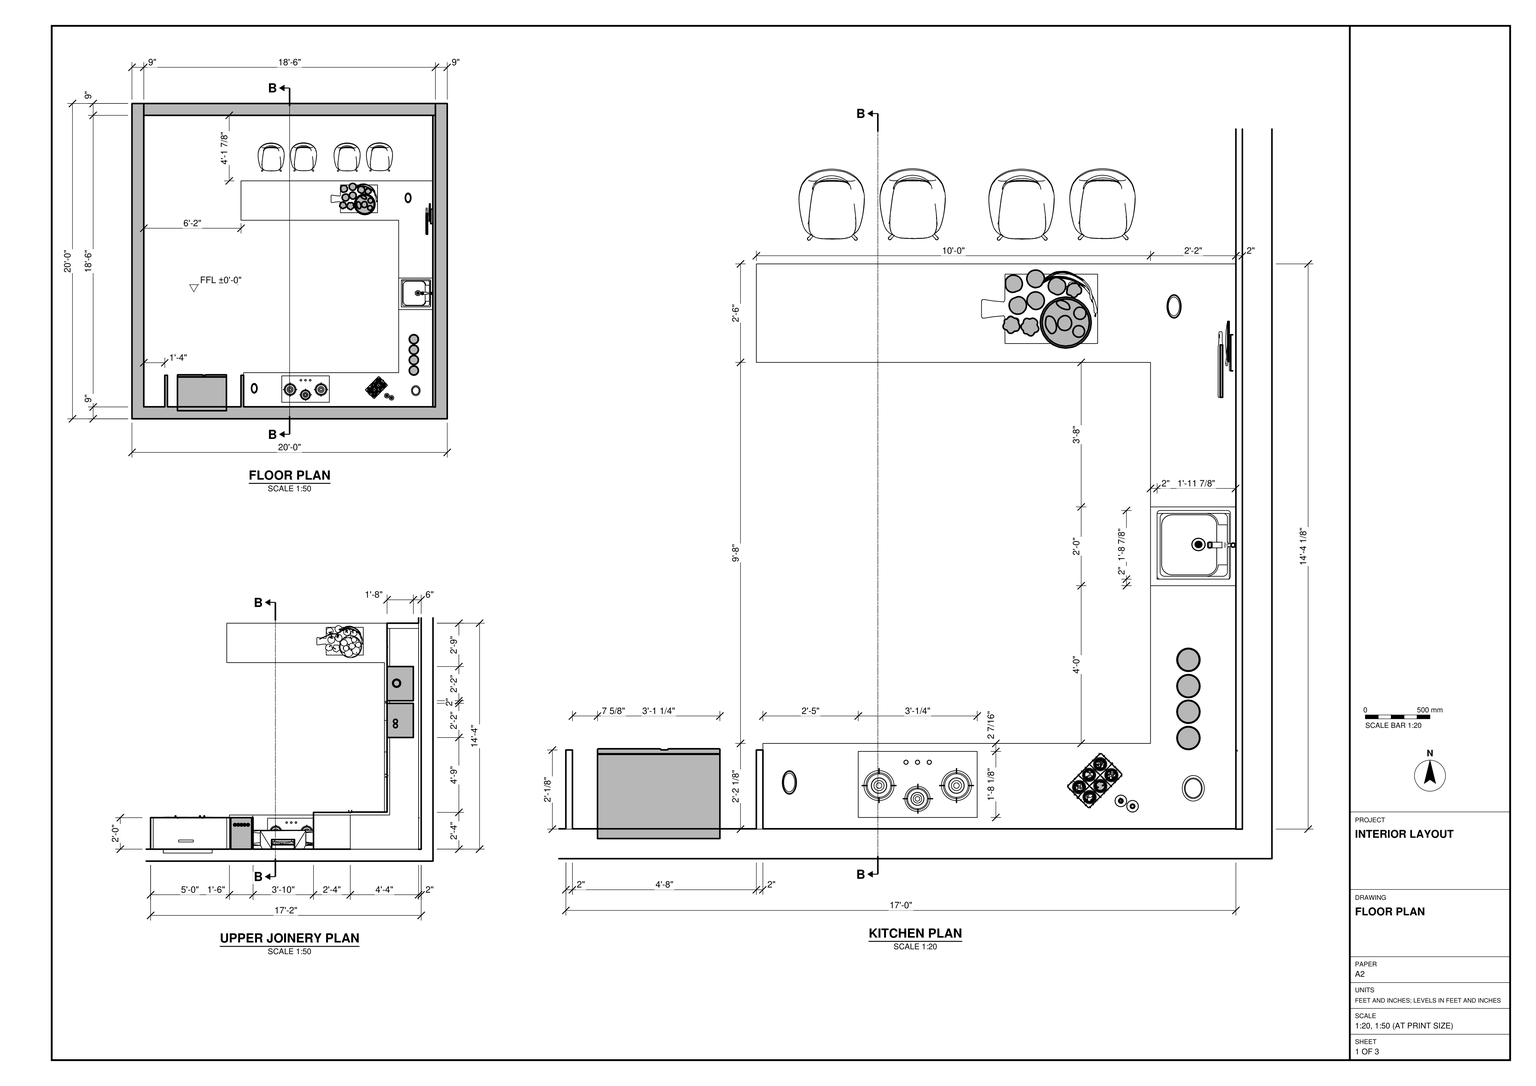
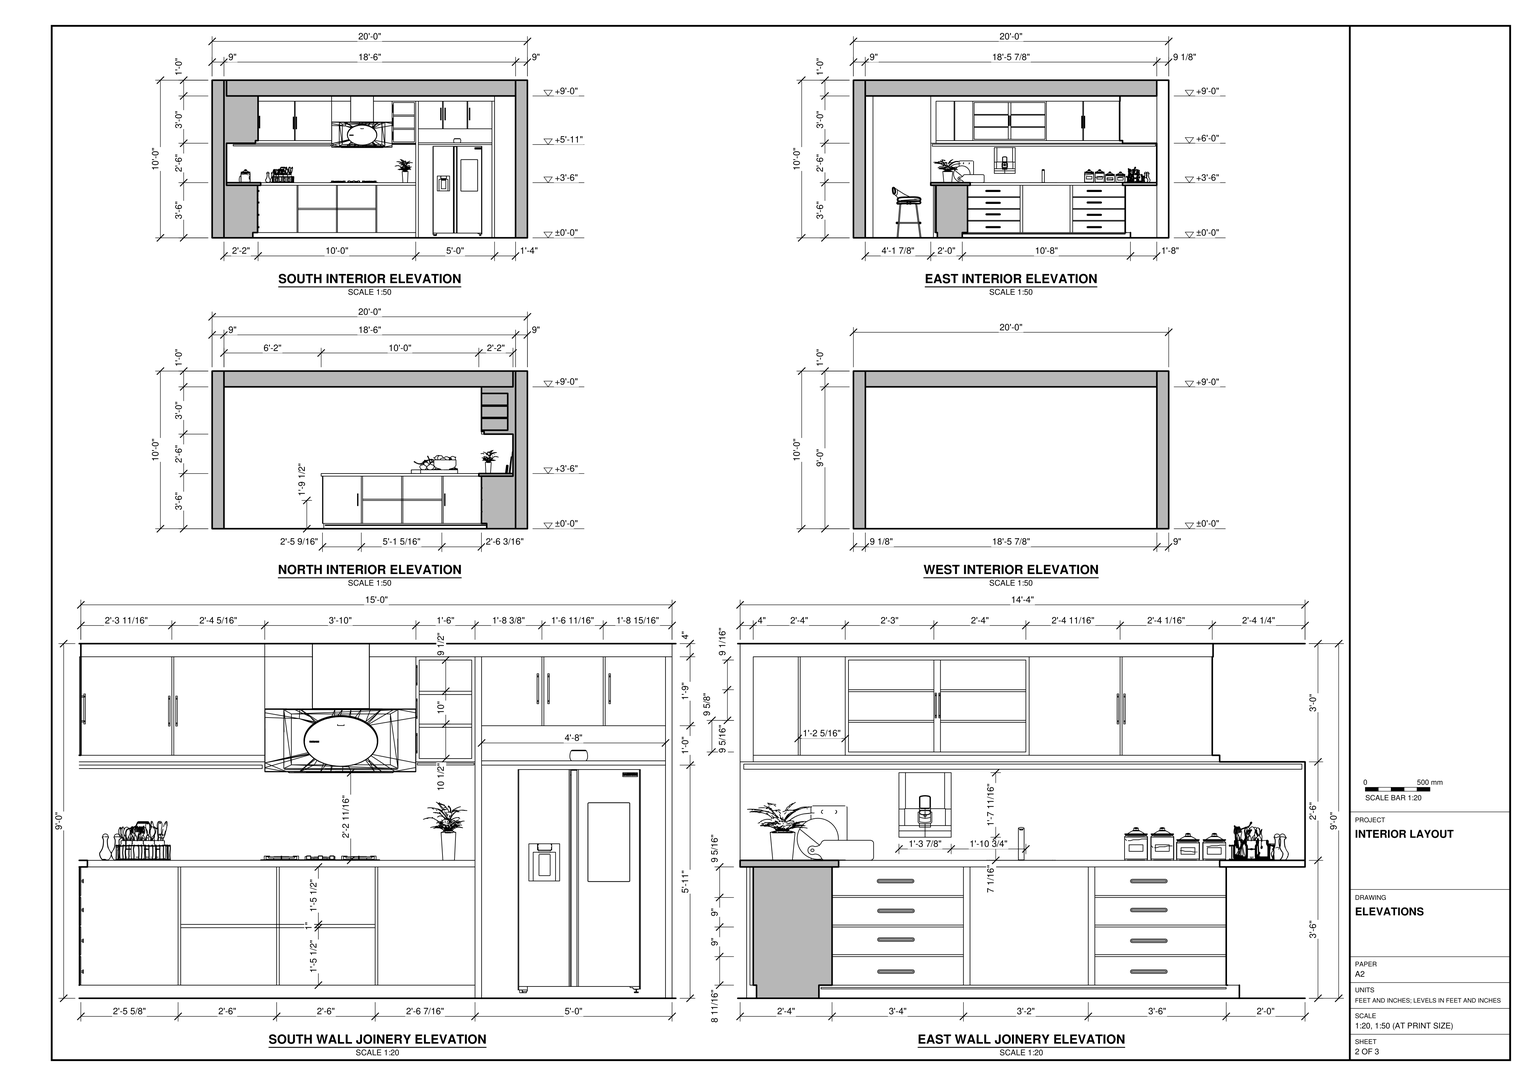
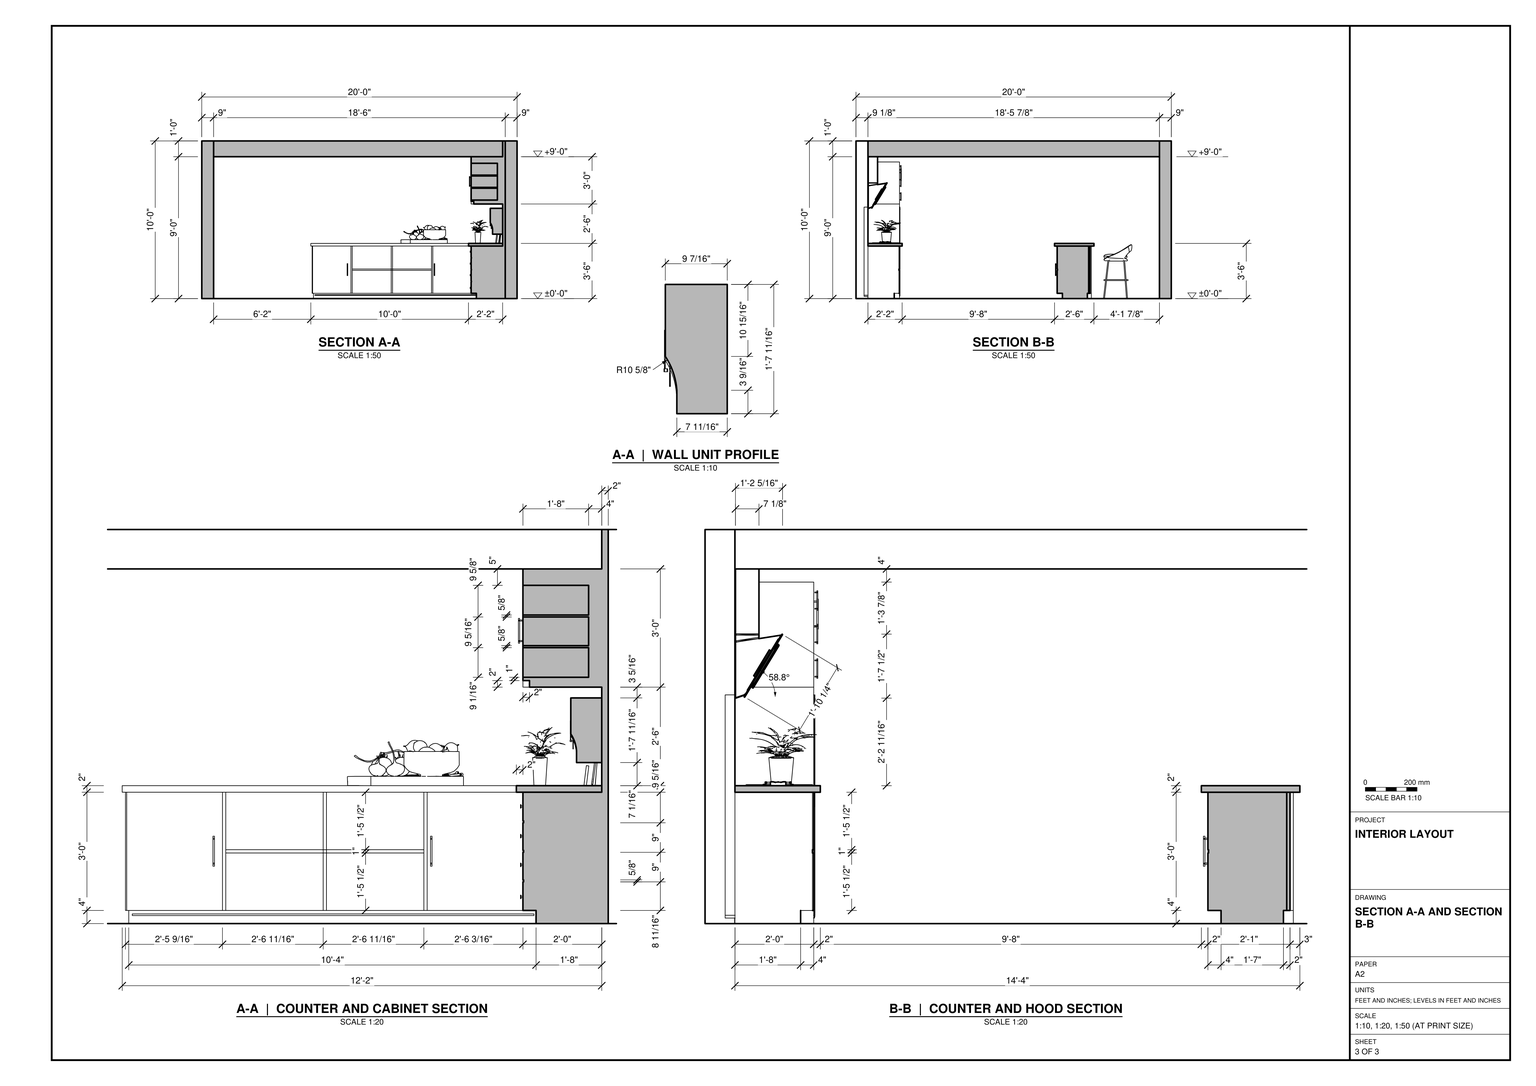
Work in feet and inches. Use task_files/diagram_01.pdf to model the kitchen in SketchUp. The overall model dimensions are 20'-0" by 20'-0" by 12'-9 13/16", with the finished floor at ±0'-0". Follow the floor plan for the 9" perimeter walls and the sections for the room enclosure, including the slab with its underside at 9'-0" above the finished floor.

Run the fitted kitchen along the south and east walls. Return the east counter into the room to form the peninsula, leaving a passage at its west end and seating on its north side. Use the joinery elevations and sections to set the counter heights, worktop edges, recessed plinths, cabinet fronts, drawer banks and upper storage. Fit the refrigerator into the tall bay, align the hood over the cooktop and set the sink into the east counter. Place the stools and counter accessories where shown. Decor and loose items, including appliances, may be any suitable library components.

Keep the shell elements and each furniture or joinery piece in separate groups or components, and use components for repeated parts. Save one SketchUp model as output_files/fitted_kitchen_with_seating_peninsula.skp.

# SketchUp Ruby script. Lengths in inches.
U = 1.inch
M = Sketchup.active_model
def pt(a) = Geom::Point3d.new(a.map { |v| v * U })
def face(e, loops, mat)
  f = e.add_face(loops[0].map { |a| pt(a) })
  loops[1..].each { |l| e.add_face(l.map { |a| pt(a) }).erase! }
  f.material = f.back_material = mat if mat
  f
end
# faces: each face lists its corners as indices into pts; further lists are holes
def faces(e, pts, list, mat = nil) = list.each { |f| face(e, (f[0].is_a?(Array) ? f : [f]).map { |l| l.map { |i| pts[i] } }, mat) }
# xy, xz, yz: faces in a plane at the given z, y or x. An outline is a flat list of corners, or four numbers for a rectangle; further outlines are holes
def ring(l) = l.size == 4 ? [[l[0], l[1]], [l[2], l[1]], [l[2], l[3]], [l[0], l[3]]] : l.each_slice(2).to_a
def flat(e, list, mat, &to3) = list.each { |f| face(e, (f[0].is_a?(Array) ? f : [f]).map { |l| ring(l).map { |u, v| to3.(u, v) } }, mat) }
def xy(e, z, list, mat = nil) = flat(e, list, mat) { |x, y| [x, y, z] }
def xz(e, y, list, mat = nil) = flat(e, list, mat) { |x, z| [x, y, z] }
def yz(e, x, list, mat = nil) = flat(e, list, mat) { |y, z| [x, y, z] }
def lines(e, pts, list) = list.each { |a, b| e.add_line(pt(pts[a]), pt(pts[b])) }
# prism: a flat outline (further loops are holes) pulled along v
def prism(e, loops, v, mat = nil)
  f = face(e, loops, mat); d = Geom::Vector3d.new(v.map { |x| x * U })
  f.pushpull(f.normal.samedirection?(d) ? d.length : -d.length)
end
def box(e, o, s, mat = nil) = prism(e, [[o, [o[0] + s[0], o[1], o[2]], [o[0] + s[0], o[1] + s[1], o[2]], [o[0], o[1] + s[1], o[2]]]], [0, 0, s[2]], mat)
def at(x, y, z, deg = 0) = Geom::Transformation.translation(pt([x, y, z])) * Geom::Transformation.rotation(ORIGIN, Z_AXIS, deg.degrees)
def axes(o, x, y, z) = Geom::Transformation.new([*x, 0, *y, 0, *z, 0, *pt(o).to_a, 1])
def part(name) = M.definitions.add(name)
# library, detail: a bought-in or finely detailed component or shape, given as its bounding box
def library(name, o, s) = part(name).tap { |d| box(d.entities, o, s) }
def detail(e, o, s) = box(e.add_group.entities, o, s)
def put(e, d, t, mat = nil) = e.add_instance(d, t).tap { |i| i.material = mat if mat }
def group(e, t, mat = nil) = e.add_group.tap { |g| g.transformation = t; g.material = mat if mat }.entities
root = M.entities
M.materials.add("Heather_PantShadow").color = [238, 181, 37]
M.materials.add("Polytec Natio Walnut").color = [132, 104, 79]
M.materials.add("SAMSUNG SMART FRIDGE").color = [78, 78, 81]
M.materials.add("[Color M09]").color = [0, 0, 0]
M.materials.add("[Translucent Glass Blue]").color = [100, 149, 237]
M.materials["[Translucent Glass Blue]"].alpha = 0.5
M.materials.add("cnwhc.com_草图联盟_1kmauOsh").color = [54, 52, 52]
M.materials.add("cnwhc.com_草图联盟_C8Y5Xp2O").color = [156, 156, 156]
M.materials["cnwhc.com_草图联盟_C8Y5Xp2O"].alpha = 0.15
M.materials.add("cnwhc.com_草图联盟_IHFcDxe1").color = [138, 151, 59]
M.materials.add("cnwhc.com_草图联盟_KNEfX85g").color = [162, 126, 87]
M.materials.add("cnwhc.com_草图联盟_QJow1Ky4").color = [144, 133, 65]
M.materials.add("cnwhc.com_草图联盟_z6N5x4Hv").color = [237, 222, 58]
c1 = library("SAMSUNG SMART FRIDGE",[0,-0.09,0],[35.91,28.28,70.08])
c2 = library("Sink with tap",[-0.11,0,0],[20.3,18.9,21.51])
c3 = part("Door Lever\#2")
detail(c3.entities,[0,0,0],[5.43,2.05,2.36])
c4 = part("Door Lever\#1")
detail(c4.entities,[0,0,0],[5.43,2.05,2.36])
c5 = part("Door Lever\#3")
detail(c5.entities,[0,0,0],[5.43,2.05,2.36])
c6 = part("200mm Half Round Handle")
xz(c6.entities,0,[[3.9375,0,3.9375,7.875,3.42,7.84,2.92,7.74,2.43,7.57,1.97,7.35,1.54,7.06,1.15,6.72,0.8125,6.33,0.53,5.91,0.3,5.44,0.13,4.96,0.03,4.45,0,3.9375,0.03,3.42,0.13,2.92,0.3,2.43,0.53,1.97,0.8125,1.54,1.15,1.15,1.54,0.8125,1.97,0.53,2.43,0.3,2.92,0.13,3.42,0.03]],"[Color M09]")
xz(c6.entities,0.12,[[3.82,0.01,3.42,0.03,2.92,0.13,2.43,0.3,1.97,0.53,1.54,0.8125,1.15,1.15,0.8125,1.54,0.53,1.97,0.3,2.43,0.13,2.92,0.03,3.42,0,3.9375,0.03,4.45,0.13,4.96,0.3,5.44,0.53,5.91,0.8125,6.33,1.15,6.72,1.54,7.06,1.97,7.35,2.43,7.57,2.92,7.74,3.42,7.84,3.82,7.87]],"[Color M09]")
xz(c6.entities,0.91,[[3.9375,0,3.82,0.01,3.82,7.87,3.9375,7.875]],"[Color M09]")
yz(c6.entities,3.82,[[0.12,0.01,0.91,7.87]],"[Color M09]")
yz(c6.entities,3.9375,[[0,0,0.91,7.875]],"[Color M09]")
p = [[3.42,0,0.03],[2.92,0,0.13],[2.92,0.12,0.13],[3.42,0.12,0.03],[3.9375,0,0],[3.82,0.12,0.01],
  [3.82,0.91,0.01],[3.9375,0.91,0],[2.43,0,0.3],[2.43,0.12,0.3],[1.97,0,0.53],[1.97,0.12,0.53],
  [1.54,0,0.8125],[1.54,0.12,0.8125],[1.15,0,1.15],[1.15,0.12,1.15],[0.8125,0,1.54],[0.8125,0.12,1.54],
  [0.53,0,1.97],[0.53,0.12,1.97],[0.3,0,2.43],[0.3,0.12,2.43],[0.13,0,2.92],[0.13,0.12,2.92],
  [0.03,0,3.42],[0.03,0.12,3.42],[0,0,3.9375],[0,0.12,3.9375],[0.03,0,4.45],[0.03,0.12,4.45],
  [0.13,0,4.96],[0.13,0.12,4.96],[0.3,0,5.44],[0.3,0.12,5.44],[0.53,0,5.91],[0.53,0.12,5.91],
  [0.8125,0,6.33],[0.8125,0.12,6.33],[1.15,0,6.72],[1.15,0.12,6.72],[1.54,0,7.06],[1.54,0.12,7.06],
  [1.97,0,7.35],[1.97,0.12,7.35],[2.43,0,7.57],[2.43,0.12,7.57],[2.92,0,7.74],[2.92,0.12,7.74],
  [3.42,0,7.84],[3.42,0.12,7.84],[3.9375,0,7.875],[3.9375,0.91,7.875],[3.82,0.91,7.87],[3.82,0.12,7.87]]
faces(c6.entities,p,[[0,1,2,3],[4,0,3,5,6,7],[1,8,9,2],[8,10,11,9],[10,12,13,11],[12,14,15,13],[14,16,17,15],[16,18,19,17],
  [18,20,21,19],[20,22,23,21],[22,24,25,23],[24,26,27,25],[26,28,29,27],[28,30,31,29],[30,32,33,31],[32,34,35,33],
  [34,36,37,35],[36,38,39,37],[38,40,41,39],[40,42,43,41],[42,44,45,43],[44,46,47,45],[46,48,49,47],[48,50,51,52,53,49]],"[Color M09]")
c7 = part("150mm Half Round Handle")
xz(c7.entities,0,[[0,0,0.12,0.01,0.12,5.9,0,5.91]],"Polytec Natio Walnut")
xz(c7.entities,0.79,[[0.12,0.01,0.39,0.03,0.76,0.1,1.13,0.22,1.48,0.4,1.8,0.61,2.09,0.86,2.34,1.16,2.56,1.48,2.73,1.82,2.85,2.1875,2.93,2.57,2.95,2.95,2.93,3.34,2.85,3.72,2.73,4.08,2.56,4.43,2.34,4.75,2.09,5.04,1.8,5.3,1.48,5.51,1.13,5.68,0.76,5.8,0.39,5.88,0.12,5.9]],"Polytec Natio Walnut")
xz(c7.entities,0.91,[[0,0,0,5.91,0.39,5.88,0.76,5.8,1.13,5.68,1.48,5.51,1.8,5.3,2.09,5.04,2.34,4.75,2.56,4.43,2.73,4.08,2.85,3.72,2.93,3.34,2.95,2.95,2.93,2.57,2.85,2.1875,2.73,1.82,2.56,1.48,2.34,1.16,2.09,0.86,1.8,0.61,1.48,0.4,1.13,0.22,0.76,0.1,0.39,0.03]],"Polytec Natio Walnut")
yz(c7.entities,0,[[0,0,0.91,5.91]],"Polytec Natio Walnut")
yz(c7.entities,0.12,[[0,0.01,0.79,5.9]],"Polytec Natio Walnut")
p = [[0,0.91,0],[0.39,0.91,0.03],[0.39,0.79,0.03],[0.12,0.79,0.01],[0.12,0,0.01],[0,0,0],
  [0.76,0.91,0.1],[0.76,0.79,0.1],[1.13,0.91,0.22],[1.13,0.79,0.22],[1.48,0.91,0.4],[1.48,0.79,0.4],
  [1.8,0.91,0.61],[1.8,0.79,0.61],[2.09,0.91,0.86],[2.09,0.79,0.86],[2.34,0.91,1.16],[2.34,0.79,1.16],
  [2.56,0.91,1.48],[2.56,0.79,1.48],[2.73,0.91,1.82],[2.73,0.79,1.82],[2.85,0.91,2.1875],[2.85,0.79,2.1875],
  [2.93,0.91,2.57],[2.93,0.79,2.57],[2.95,0.91,2.95],[2.95,0.79,2.95],[2.93,0.91,3.34],[2.93,0.79,3.34],
  [2.85,0.91,3.72],[2.85,0.79,3.72],[2.73,0.91,4.08],[2.73,0.79,4.08],[2.56,0.91,4.43],[2.56,0.79,4.43],
  [2.34,0.91,4.75],[2.34,0.79,4.75],[2.09,0.91,5.04],[2.09,0.79,5.04],[1.8,0.91,5.3],[1.8,0.79,5.3],
  [1.48,0.91,5.51],[1.48,0.79,5.51],[1.13,0.91,5.68],[1.13,0.79,5.68],[0.76,0.91,5.8],[0.76,0.79,5.8],
  [0.39,0.91,5.88],[0.39,0.79,5.88],[0,0.91,5.91],[0,0,5.91],[0.12,0,5.9],[0.12,0.79,5.9]]
faces(c7.entities,p,[[0,1,2,3,4,5],[1,6,7,2],[6,8,9,7],[8,10,11,9],[10,12,13,11],[12,14,15,13],[14,16,17,15],[16,18,19,17],
  [18,20,21,19],[20,22,23,21],[22,24,25,23],[24,26,27,25],[26,28,29,27],[28,30,31,29],[30,32,33,31],[32,34,35,33],
  [34,36,37,35],[36,38,39,37],[38,40,41,39],[40,42,43,41],[42,44,45,43],[44,46,47,45],[46,48,49,47],[48,50,51,52,53,49]],"Polytec Natio Walnut")
c8 = part("148mm Black Satin Pull\#1")
prism(c8.entities,[[[5.83,0.12,0.5],[5.83,0.16,0.49],[5.83,0.16,0],[5.83,0.31,0],[5.83,0.31,0.49],[5.83,0.35,0.5],[5.83,0.4,0.54],[5.83,0.44,0.59],[5.83,0.46,0.65],[5.83,0.47,0.71],[5.83,0.46,0.77],[5.83,0.44,0.83],[5.83,0.4,0.875],[5.83,0.35,0.91],[5.83,0.3,0.9375],[5.83,0.24,0.94],[5.83,0.18,0.9375],[5.83,0.12,0.91],[5.83,0.07,0.875],[5.83,0.03,0.83],[5.83,0.01,0.77],[5.83,0,0.71],[5.83,0.01,0.65],[5.83,0.03,0.59],[5.83,0.07,0.54]]],[-5.83,0,0],"[Color M09]")
p = [[5.83,0.16,0.59],[0,0.16,0.59],[5.83,0.31,0.59],[0,0.31,0.59]]
lines(c8.entities,p,[[0,1],[2,3]])
c9 = part("232mm Slimline Handle\#1")
detail(c9.entities,[0,0,0],[9.13,0.47,1.38])
c10 = part("232mm Slimline Handle")
detail(c10.entities,[0,0,0],[9.13,0.47,1.38])
c11 = library("Bosch Stove",[0,0,0],[36.22,20.12,1.38])
c12 = library("Plant",[-15.17,-14.95,0],[35.27,31.45,46.14])
c13 = library("Potted plant",[0.24,-1.94,0],[14.49,14.49,6.23])
c14 = library("78970097",[-100,-100,0],[200,200,30])
c15 = library("78970100",[-75,-75,0],[150,150,60])
c16 = library("Food+(14)",[-17.72,-12.23,0],[35.37,24.44,13.82])
c17 = library("Chopping baords",[-2.18,0,-3.9],[25.44,5.42,20.47])
c18 = library("Chimney",[0,-14.34,0],[33.95,14.34,33.72])
c19 = library("WEST_ELM_Orb_Bar_Counter_Stools",[-10.93,-22.29,0],[21.86,44.58,41.07])
c20 = library("Lg+Water+purifier (1)",[0,2.4,0],[10.83,14.37,19.92])
c21 = part("Group\#7")
box(c21.entities,[0,0,0],[1,1,36])
c22 = part("Group\#346")
detail(c22.entities,[0,0,0],[11.18,0.75,1.1])
c23 = library("Group\#35",[-453.95,-270.9,-0.08],[243.89,243.63,216.82])
c24 = library("Group\#116",[-376.9,120.94,-0.1],[107.79,107.8,326.37])
c25 = library("Group\#113",[0.46,121.12,-0.1],[106.94,106.94,338.14])
c26 = library("Group\#117",[-504.125,120.57,-0.1],[108.2,108.21,338.13])
c27 = library("Group\#115",[-254.81,120.48,-0.6],[108.21,108.21,334.5])
c28 = library("Group\#114",[-133.01,121.19,-0.1],[106.95,106.95,324.89])
c29 = library("Group\#130",[-198.8,84.74,613.85],[84,84,172.39])
c30 = library("Group\#129",[-105.26,84.74,613.85],[84,84,172.39])
c31 = library("Group\#123",[-15.73,84.74,613.85],[84,84,172.39])
c32 = library("Group\#132",[-374.05,84.21,613.65],[72.44,72.44,111.8])
c33 = library("Group\#131",[-289.4,84.22,613.65],[72.44,72.43,111.8])
c34 = library("Group\#133",[-462.66,84.21,613.65],[72.44,72.44,111.8])
c35 = library("Group77\#2",[-35,-35,0],[70,70,205])
c36 = library("Group76\#2",[-35,-35,0],[70,70,205])
c37 = library("Group\#260",[0,0,0],[30.82,7.02,10])
c38 = library("Group\#48",[198.24,-475.92,149.53],[39.78,40.55,40.71])
c39 = library("Group\#49",[-248.47,-468.28,0.39],[392.05,393.05,278.56])
c40 = library("Group\#50",[-141.57,-278.65,11.2],[96.36,96.33,131.41])
c41 = library("Group\#51",[-62.08,-202.43,11.2],[96.04,96.07,131.41])
c42 = library("Group\#43",[91.875,-459.8125,1.36],[84.84,84.82,167.94])
c43 = library("Group\#44",[93.63,-458.06,3.28],[81.33,81.31,90.04])
c44 = library("Group\#45",[114.46,-437.1875,150.05],[39.68,39.57,39.67])
c45 = library("Group\#42",[118.34,-437.05,68.8],[33.09,42.97,27.32])
c46 = library("Group\#46",[177.52,-496.26,3.28],[81.21,81.23,127.94])
c47 = library("Group\#47",[175.77,-498.01,1.36],[84.71,84.74,167.94])
c48 = library("Group\#61",[-142.58,-458.38,19.87],[79.66,135.74,256])
c49 = library("Group\#55",[8.05,-292.87,22.71],[116.19,111.01,218.49])
c50 = library("Group\#58",[-64.19,-232.55,22.9],[102.65,128.29,224.14])
c51 = library("Group\#60",[-138.35,-437.94,11.2],[96.49,96.52,131.41])
c52 = library("Group\#59",[-225.25,-376.69,19.19],[116.52,116.69,261.73])
c53 = library("Group\#56",[-64.85,-368.89,23],[127.95,108.9,222.0625])
c54 = library("Group\#57",[-143.92,-281.53,22.82],[119.68,105.06,218.38])
c55 = library("Group\#53",[-213.25,-366.61,11.2],[96.18,96.15,131.41])
c56 = library("Group\#52",[18.13,-280.93,11.2],[96.51,96.54,131.41])
c57 = library("Group\#54",[-61.03,-358.93,11.2],[96.54,96.51,131.41])
c58 = part("Fitted kitchen interior")
xy(c58.entities,0,[[220.03,0,222,0,222,222,220.03,222,220.03,170.125,218.03,170.125,218.03,167.125,78,167.125,78,170.125,76,170.125,76,148.125,200.03,148.125,200.03,24.1,220.03,24.1],[0,0.1,16,0.1,16,24.1,18,24.1,18,0.1,74,0.1,74,24.1,76,24.1,76,20.1,200.03,20.1,200.03,148.125,76,148.125,76,170.125,78,170.125,78,167.125,218.03,167.125,218.03,170.125,220.03,170.125,220.03,222,0,222]])
xy(c58.entities,4,[[196.03,20.1,200.03,23.73],[196.03,23.73,200.03,24.1],[196.03,24.1,196.03,64.11,196.43,64.11,196.43,66.11,196.03,66.11,196.03,102.12,196.23,102.12,196.23,104.12,196.03,104.12,196.03,148.125,200.03,148.125,200.03,24.1],[75.375,144.125,75.375,145.125,75,145.125,75,148.125,196.03,148.125,196.03,144.125,166.86,144.125,166.86,144.33,165.86,144.33,165.86,144.125,136.2,144.125,136.2,144.33,135.2,144.33,135.2,144.125,105.54,144.125,105.54,144.33,104.54,144.33,104.54,144.125],[75,148.125,76,166.59],
  [[78,167.125,218.03,168.125],[78.64,167.51,217.95,167.88]]])
xy(c58.entities,4,[[81.15,23.73,105.61,24.1],[105.61,23.73,106.41,24.1],[106.41,23.73,135.61,24.1],[135.61,23.73,136.41,24.1],[136.41,23.73,196.03,24.1],
  [200.03,23.73,220.46,24.1],[78.64,167.51,217.95,167.88]],"Heather_PantShadow")
xy(c58.entities,12.7,[[196.03,24.1,196.23,64.11],[196.03,104.12,196.23,144.125]])
xy(c58.entities,13.3,[[196.03,24.1,196.23,64.11],[196.03,104.12,196.23,144.125]])
xy(c58.entities,21.5,[[106.41,23.7,135.61,24.1],[136.41,23.7,165.62,24.1],[105.54,144.125,135.2,144.33],[136.2,144.125,165.86,144.33]])
xy(c58.entities,21.5,[[135.61,23.7,136.41,24.1]],"[Color M09]")
xy(c58.entities,21.7,[[196.03,24.1,196.23,64.11],[196.03,104.12,196.23,144.125]])
xy(c58.entities,22.3,[[196.03,24.1,196.23,64.11],[196.03,104.12,196.23,144.125]])
xy(c58.entities,22.5,[[106.41,23.7,135.61,24.1],[136.41,23.7,165.62,24.1],[105.54,144.125,135.2,144.33],[136.2,144.125,165.86,144.33]])
xy(c58.entities,22.5,[[135.61,23.7,136.41,24.1],[135.2,144.33,136.2,144.53]],"[Color M09]")
xy(c58.entities,30.7,[[196.03,24.1,196.23,64.11],[196.03,104.12,196.23,144.125]])
xy(c58.entities,31.3,[[196.03,24.1,196.23,64.11],[196.03,104.12,196.23,144.125]])
xy(c58.entities,40,[[[76,0.1,76,24.1,105.61,24.1,105.61,23.7,106.41,23.7,106.41,24.1,135.61,24.1,135.61,23.7,136.41,23.7,136.41,24.1,165.62,24.1,165.62,23.7,166.42,23.7,166.42,24.1,196.03,24.1,196.03,64.11,196.43,64.11,196.43,66.11,196.03,66.11,196.03,76.125,218.03,76.125,218.03,96.125,196.03,96.125,196.03,102.12,196.23,102.12,196.23,104.12,196.03,104.12,196.03,142.125,74,142.125,74,172.125,218.03,172.125,218.03,170.125,220.03,170.125,220.03,0.1],[75.33,170.58,217.64,171.15]],[105.61,23.7,105.61,24.1,76,24.1,76,26.1,194.03,26.1,194.03,24.1,166.42,24.1,166.42,23.7,165.62,23.7,165.62,24.1,136.41,24.1,136.41,23.7,135.61,23.7,135.61,24.1,106.41,24.1,106.41,23.7],[194.03,24.1,194.03,142.125,196.03,142.125,196.03,104.12,196.23,104.12,196.23,102.12,196.03,102.12,196.03,66.11,196.43,66.11,196.43,64.11,196.03,64.11,196.03,24.1],[104.54,144.125,105.54,144.33],[135.2,144.125,136.2,144.53],
  [165.86,144.125,166.86,144.33],[218.03,170.125,220.03,172.125]])
xy(c58.entities,40,[[75.33,170.58,217.64,171.15]],"Heather_PantShadow")
xy(c58.entities,42,[[76,0.1,220.03,0.1,220.03,74.125,194.03,74.125,194.03,26.1,76,26.1],[[194.03,74.125,220.03,98.125],[196.03,76.125,218.03,96.125]],[194.03,98.125,220.03,98.125,220.03,172.125,74,172.125,74,142.125,194.03,142.125]])
xy(c58.entities,71,[[18,0.1,74,24.1]])
xy(c58.entities,72,[[76,0.1,94,24.1],[140.03,0.1,168.03,26.1],[168.03,0.1,168.03,26.1,198.03,26.1,198.03,168.125,220.03,168.125,220.03,0.1],[196.03,168.125,220.03,172.125]])
xy(c58.entities,72.3125,[[18,0.1,74,24.1]])
xy(c58.entities,73,[[77,0.1,93,24.1]])
xy(c58.entities,74,[[140.03,26.1,140.03,28.1,167.73,28.1,167.73,27.9,168.32,27.9,168.32,28.35,196.03,28.35,196.03,55.81,196.43,55.81,196.43,56.41,196.03,56.41,196.03,153.82,196.23,153.82,196.23,154.42,196.03,154.42,196.03,168.125,198.03,168.125,198.03,26.1]])
xy(c58.entities,75,[[196.03,85.11,216.03,111.12],[196.03,113.12,216.03,139.12]])
xy(c58.entities,82.5,[[[77,0.1,93,24.1],[77.08,0.54,92.83,1.61]]])
xy(c58.entities,82.5,[[77.08,0.54,92.83,1.61]],"Heather_PantShadow")
xy(c58.entities,83,[[[18,0.1,18,24.1,36.37,24.1,36.37,23.9,36.97,23.9,36.97,24.1,55.03,24.1,55.03,23.9,55.63,23.9,55.63,24.1,74,24.1,74,0.1],[37.34,5.58,48.53,7.08]]])
xy(c58.entities,83,[[37.34,5.58,48.53,7.08]],"Heather_PantShadow")
xy(c58.entities,83.5,[[77,0.1,93,24.1]])
xy(c58.entities,84.03,[[[196.03,85.11,216.03,111.12],[209.98,85.6875,213.04,110.6875]],[[196.03,113.12,216.03,139.12],[209.98,113.6875,213.04,138.6875]]])
xy(c58.entities,84.03,[[209.98,85.6875,213.04,110.6875],[209.98,113.6875,213.04,138.6875]],"Heather_PantShadow")
xy(c58.entities,84.63,[[196.03,85.11,216.03,111.12],[196.03,113.12,216.03,139.12]])
xy(c58.entities,92.5,[[[77,0.1,93,24.1],[77.08,0.54,92.83,1.61]]])
xy(c58.entities,92.5,[[77.08,0.54,92.83,1.61]],"Heather_PantShadow")
xy(c58.entities,93.37,[[[196.03,85.11,216.03,111.12],[209.98,85.625,213.04,110.625]],[[196.03,113.12,216.03,139.12],[209.98,113.6875,213.04,138.6875]]])
xy(c58.entities,93.37,[[209.98,85.625,213.04,110.625],[209.98,113.6875,213.04,138.6875]],"Heather_PantShadow")
xy(c58.entities,93.5,[[77,0.1,93,24.1]])
xy(c58.entities,93.97,[[196.03,85.11,216.03,111.12],[196.03,113.12,216.03,139.12]])
xy(c58.entities,103,[[[77,0.1,93,24.1],[77.08,0.54,92.83,1.61]],[[196.03,85.11,216.03,111.12],[209.98,85.6875,213.04,110.6875]],[[196.03,113.12,216.03,139.12],[209.98,113.6875,213.04,138.6875]]])
xy(c58.entities,103,[[77.08,0.54,92.83,1.61],[209.98,85.6875,213.04,110.6875],[209.98,113.6875,213.04,138.6875]],"Heather_PantShadow")
xy(c58.entities,104,[[16,0.1,94,0.1,94,24.1,55.63,24.1,55.63,23.9,55.03,23.9,55.03,24.1,36.97,24.1,36.97,23.9,36.37,23.9,36.37,24.1,16,24.1],[167.73,27.9,168.32,28.1],[168.32,28.1,196.03,28.35],[196.03,55.81,196.43,56.41],[196.03,153.82,196.23,154.42]])
xy(c58.entities,108,[[140.03,0.1,220.03,0.1,220.03,172.125,196.03,172.125,196.03,28.1,140.03,28.1]])
xy(c58.entities,120,[[0,0,220.03,0.1],[220.03,0,222,222]])
xz(c58.entities,0,[[220.03,0,222,120]])
xz(c58.entities,0.1,[[0,0,0,120,220.03,120,220.03,108,16,108,16,0],[18,0,74,71],[76,40,220.03,42],[[76,42,76,72,94,72,94,104,140.03,104,140.03,72,220.03,72,220.03,42],[140.79,69.95,214.98,71.02],[76.29,71.06,93.6,71.62]],[16,71,18,74.3125],
  [18,71,74,72.3125],[74,71,76,84],[140.03,72,168.03,108],[18,72.3125,74,83],[77,73,93,82.5],
  [16,74.3125,16,84,74,84,74,83,18,83,18,74.3125],[77,83.5,93,92.5],[16,84,74,104],[74,84,76,104],[77,93.5,93,103],
  [16,104,140.03,108]])
xz(c58.entities,0.1,[[140.79,69.95,214.98,71.02],[76.29,71.06,93.6,71.62]],"Heather_PantShadow")
xz(c58.entities,20.1,[[76,0,200.03,4]])
xz(c58.entities,23.7,[[105.61,4,106.41,40],[135.61,4,136.41,21.5],[106.41,21.5,135.61,22.5],[136.41,21.5,165.62,22.5],[135.61,22.5,136.41,40]],"[Color M09]")
xz(c58.entities,23.9,[[36.37,83,36.97,104],[55.03,83,55.63,104]],"[Color M09]")
xz(c58.entities,24.1,[[16,0,18,104],[74,0,76,104],[76,4,105.61,40],[106.41,4,135.61,21.5],[136.41,4,165.62,21.5],
  [166.42,4,166.42,40,196.03,40,196.03,31.3,196.23,31.3,196.23,30.7,196.03,30.7,196.03,22.3,196.23,22.3,196.23,21.7,196.03,21.7,196.03,13.3,196.23,13.3,196.23,12.7,196.03,12.7,196.03,4],[106.41,22.5,135.61,40],[136.41,22.5,165.62,40],[18,71,74,72.3125],[18,83,36.37,104],
  [36.97,83,55.03,104],[55.63,83,74,104]])
xz(c58.entities,24.1,[[135.61,21.5,136.41,22.5],[[76,72,94,104],[77,73,93,103]],[77,82.5,93,83.5],[77,92.5,93,93.5]],"[Color M09]")
xz(c58.entities,24.1,[[77,73,93,82.5],[77,83.5,93,92.5],[77,93.5,93,103]],"[Translucent Glass Blue]")
xz(c58.entities,26.1,[[76,40,194.03,42],[140.03,72,198.03,74]])
xz(c58.entities,27.9,[[167.73,74,168.32,104]],"[Color M09]")
xz(c58.entities,28.1,[[140.03,74,167.73,104],[140.03,104,196.03,108]])
xz(c58.entities,28.35,[[168.32,74,196.03,104]])
xz(c58.entities,55.81,[[196.03,74,196.43,104]])
xz(c58.entities,56.41,[[196.03,74,196.43,104]])
xz(c58.entities,64.11,[[196.03,4,196.43,12.7],[196.23,12.7,196.43,13.3],[196.03,13.3,196.43,21.7],[196.23,21.7,196.43,22.3],[196.03,22.3,196.43,30.7],
  [196.23,30.7,196.43,31.3],[196.03,31.3,196.43,40]])
xz(c58.entities,66.11,[[196.03,4,196.43,12.7],[196.03,12.7,196.43,13.3],[196.03,13.3,196.43,21.7],[196.03,21.7,196.43,22.3],[196.03,22.3,196.43,30.7],
  [196.03,30.7,196.43,31.3],[196.03,31.3,196.43,40]])
xz(c58.entities,76.125,[[196.03,40,218.03,42]])
xz(c58.entities,85.11,[[196.03,75,216.03,84.03],[196.03,84.63,216.03,93.37],[196.03,93.97,216.03,103]])
xz(c58.entities,96.125,[[196.03,40,218.03,42]])
xz(c58.entities,102.12,[[196.03,4,196.23,12.7],[196.03,12.7,196.23,13.3],[196.03,13.3,196.23,21.7],[196.03,21.7,196.23,22.3],[196.03,22.3,196.23,30.7],
  [196.03,30.7,196.23,31.3],[196.03,31.3,196.23,40]])
xz(c58.entities,104.12,[[196.03,4,196.23,12.7],[196.03,13.3,196.23,21.7],[196.03,22.3,196.23,30.7],[196.03,31.3,196.23,40]])
xz(c58.entities,111.12,[[196.03,75,216.03,84.03],[196.03,84.63,216.03,93.37],[196.03,93.97,216.03,103]])
xz(c58.entities,113.12,[[196.03,75,216.03,84.03],[196.03,84.63,216.03,93.37],[196.03,93.97,216.03,103]])
xz(c58.entities,139.12,[[196.03,75,216.03,84.03],[196.03,84.63,216.03,93.37],[196.03,93.97,216.03,103]])
xz(c58.entities,142.125,[[74,40,194.03,42]])
xz(c58.entities,144.125,[[75.375,4,104.54,40],[105.54,4,135.2,21.5],[136.2,4,165.86,21.5],[166.86,4,196.03,40],[196.03,12.7,196.23,13.3],
  [196.03,21.7,196.23,22.3],[105.54,22.5,135.2,40],[136.2,22.5,165.86,40],[196.03,30.7,196.23,31.3]])
xz(c58.entities,144.33,[[104.54,4,105.54,40],[165.86,4,166.86,40]])
xz(c58.entities,144.33,[[135.2,4,136.2,21.5],[105.54,21.5,135.2,22.5],[135.2,21.5,136.2,22.5],[136.2,21.5,165.86,22.5]],"[Color M09]")
xz(c58.entities,144.53,[[135.2,22.5,136.2,40]],"[Color M09]")
xz(c58.entities,145.125,[[75,4,75.375,40]])
xz(c58.entities,148.125,[[[76,0,200.03,4],[77.07,2.44,199.38,2.94]]])
xz(c58.entities,148.125,[[77.07,2.44,199.38,2.94]],"Heather_PantShadow")
xz(c58.entities,153.82,[[196.03,74,196.23,104]])
xz(c58.entities,154.42,[[196.03,74,196.23,104]])
xz(c58.entities,166.59,[[75,4,76,40]])
xz(c58.entities,167.125,[[78,0,218.03,4]])
xz(c58.entities,168.125,[[79,4,218.03,40],[196.03,72,198.03,74]])
xz(c58.entities,170.125,[[76,0,78,40],[218.03,0,220.03,40]])
xz(c58.entities,172.125,[[74,40,220.03,42],[196.03,72,220.03,74],[196.03,74,220.03,108]])
xz(c58.entities,222,[[220.03,0,222,120]])
yz(c58.entities,0,[[0,0,0.1,120]])
yz(c58.entities,16,[[0.1,0,24.1,104]])
yz(c58.entities,18,[[0.1,0,24.1,71],[0.1,71,4.1,72.3125],[4.1,71,24.1,72.3125],[0.1,72.3125,24.1,83]])
yz(c58.entities,36.37,[[23.9,83,24.1,84],[23.9,84,24.1,104]])
yz(c58.entities,36.97,[[23.9,83,24.1,84],[23.9,84,24.1,104]])
yz(c58.entities,55.03,[[23.9,83,24.1,84],[23.9,84,24.1,104]])
yz(c58.entities,55.63,[[23.9,83,24.1,84],[23.9,84,24.1,104]])
yz(c58.entities,74,[[0.1,0,24.1,71],[142.125,40,172.125,42],[0.1,71,4.1,72.3125],[4.1,71,24.1,72.3125],[0.1,72.3125,24.1,83]])
yz(c58.entities,75,[[145.125,4,166.59,40]])
yz(c58.entities,75.375,[[144.125,4,145.125,40]])
yz(c58.entities,76,[[20.1,0,24.1,4],[148.125,0,148.125,4,166.59,4,166.59,40,170.125,40,170.125,0],[0.1,40,24.1,42],[24.1,40,26.1,42],[0.1,42,24.1,72],
  [0.1,72,24.1,84]])
yz(c58.entities,77,[[0.1,73,24.1,82.5],[0.1,83.5,24.1,92.5],[0.1,93.5,24.1,103]])
yz(c58.entities,78,[[167.125,0,170.125,4],[168.125,4,170.125,40]])
yz(c58.entities,93,[[0.1,73,24.1,82.5],[0.1,83.5,24.1,92.5],[0.1,93.5,24.1,103]])
yz(c58.entities,94,[[0.1,72,24.1,104]])
yz(c58.entities,104.54,[[144.125,4,144.33,21.5],[144.125,21.5,144.33,22.5],[144.125,22.5,144.33,40]])
yz(c58.entities,105.54,[[144.125,4,144.33,21.5],[144.125,22.5,144.33,40]])
yz(c58.entities,105.61,[[23.7,4,24.1,21.5],[23.7,21.5,24.1,22.5],[23.7,22.5,24.1,40]])
yz(c58.entities,106.41,[[23.7,4,24.1,21.5],[23.7,22.5,24.1,40]])
yz(c58.entities,135.2,[[144.125,4,144.33,21.5],[144.125,22.5,144.53,40]])
yz(c58.entities,135.61,[[23.7,4,24.1,21.5],[23.7,22.5,24.1,40]])
yz(c58.entities,135.61,[[23.7,21.5,24.1,22.5]],"[Color M09]")
yz(c58.entities,136.2,[[144.125,4,144.33,21.5],[144.125,22.5,144.53,40]])
yz(c58.entities,136.41,[[23.7,4,24.1,21.5],[23.7,22.5,24.1,40]])
yz(c58.entities,136.41,[[23.7,21.5,24.1,22.5]],"[Color M09]")
yz(c58.entities,140.03,[[0.1,72,0.1,104,28.1,104,28.1,74,26.1,74,26.1,72],[0.1,104,28.1,108]])
yz(c58.entities,165.62,[[23.7,22.5,24.1,40]])
yz(c58.entities,165.86,[[144.125,4,144.33,21.5],[144.125,22.5,144.33,40]])
yz(c58.entities,166.42,[[23.7,21.5,24.1,22.5],[23.7,22.5,24.1,40]])
yz(c58.entities,166.86,[[144.125,4,144.33,21.5],[144.125,21.5,144.33,22.5],[144.125,22.5,144.33,40]])
yz(c58.entities,167.73,[[27.9,74,28.1,104]])
yz(c58.entities,168.32,[[27.9,74,28.35,104]])
yz(c58.entities,194.03,[[26.1,40,142.125,42]])
yz(c58.entities,196.03,[[24.1,4,64.11,12.7],[66.11,4,102.12,40],[104.12,4,144.125,12.7],[24.1,13.3,64.11,21.7],[104.12,13.3,144.125,21.7],
  [24.1,22.3,64.11,30.7],[104.12,22.3,144.125,30.7],[24.1,31.3,64.11,40],[104.12,31.3,144.125,40],[76.125,40,96.125,42],
  [168.125,72,168.125,104,28.1,104,28.1,108,172.125,108,172.125,72],[28.35,74,55.81,104],[56.41,74,84.11,104],[140.12,74,153.82,104],[154.42,74,168.125,104]])
yz(c58.entities,196.03,[[[84.11,74,140.12,104],[85.11,75,139.12,103]],[111.12,75,113.12,103],[85.11,84.03,111.12,84.63],[113.12,84.03,139.12,84.63],[85.11,93.37,111.12,93.97],
  [113.12,93.37,139.12,93.97]],"[Color M09]")
yz(c58.entities,196.03,[[85.11,75,111.12,84.03],[113.12,75,139.12,84.03],[85.11,84.63,111.12,93.37],[113.12,84.63,139.12,93.37],[85.11,93.97,111.12,103],
  [113.12,93.97,139.12,103]],"[Translucent Glass Blue]")
yz(c58.entities,196.23,[[102.12,4,104.12,40],[24.1,12.7,64.11,13.3],[104.12,12.7,144.125,13.3],[24.1,21.7,64.11,22.3],[104.12,21.7,144.125,22.3],
  [24.1,30.7,64.11,31.3],[104.12,30.7,144.125,31.3],[153.82,74,154.42,104]],"[Color M09]")
yz(c58.entities,196.43,[[64.11,4,66.11,40],[55.81,74,56.41,104]],"[Color M09]")
yz(c58.entities,198.03,[[26.1,72,168.125,74]])
yz(c58.entities,200.03,[[[20.1,0,148.125,4],[24.11,2.85,147.49,3.29]]])
yz(c58.entities,200.03,[[24.11,2.85,147.49,3.29]],"Heather_PantShadow")
yz(c58.entities,216.03,[[85.11,75,111.12,84.03],[113.12,75,139.12,84.03],[85.11,84.63,111.12,93.37],[113.12,84.63,139.12,93.37],[85.11,93.97,111.12,103],
  [113.12,93.97,139.12,103]])
yz(c58.entities,218.03,[[167.125,0,167.125,4,168.125,4,168.125,40,170.125,40,170.125,0],[76.125,40,96.125,42]])
yz(c58.entities,220.03,[[216.125,0,216.125,108,0.1,108,0.1,120,222,120,222,0],[170.125,0,170.125,40,172.125,40,172.125,108,216.125,108,216.125,0],[0.1,40,172.125,42],[[0.1,42,172.125,72],[1.07,69.75,171.01,71.3125]]])
yz(c58.entities,220.03,[[1.07,69.75,171.01,71.3125]],"Heather_PantShadow")
yz(c58.entities,222,[[0,0,222,120]])
p = [[74,0.1,84],[74,24.1,84],[165.62,23.7,4],[165.62,23.7,21.5],[166.42,23.7,4],[166.42,23.7,21.5]]
lines(c58.entities,p,[[0,1],[2,3],[4,5]])
detail(c58.entities,[93.6,24.4375,85.1875],[0.31,0.9,5.98])
detail(c58.entities,[93.6,24.4375,74.6875],[0.31,0.9,5.98])
detail(c58.entities,[93.6,24.4375,95.375],[0.31,0.9,5.98])
put(c58.entities,c1,axes([62.9,24.47,1.68],[-1.0379,0,0],[0,-0.97,0],[0,0,0.97]))
put(c58.entities,c2,axes([219.9,97.03,33.76],[-1.18221,0,0],[0,-1.10604,0],[0,0,0.85]))
put(c58.entities,c3,at(217.98,127.45,142.5,-90))
put(c58.entities,c4,at(217.98,127.45,149.71,-90))
put(c58.entities,c5,at(217.98,127.45,146.11,-90))
put(c58.entities,c6,axes([219.12,133.57,146.55],[0,1,0],[1,0,0],[0,0,-1]))
put(c58.entities,c7,axes([220.03,141.9,145.32],[0,-1,0],[-1,0,0],[0,0,-1]))
put(c58.entities,c8,axes([220.03,135.36,153.3],[0,-1,0],[0,0,1],[-1,0,0]))
put(c58.entities,c9,axes([195.79,111.23,85.39],[0,0,0.8265],[0,0.8265,0],[-0.8265,0,0]),"[Color M09]")
put(c58.entities,c10,axes([168.86,28.35,82.9],[0,0,1],[1,0,0],[0,1,0]),"[Color M09]")
put(c58.entities,c10,axes([196.03,54.84,83.54],[0,0,1],[0,1,0],[-1,0,0]),"[Color M09]")
put(c58.entities,c10,axes([166.65,28.35,82.9],[0,0,1],[1,0,0],[0,1,0]),"[Color M09]")
put(c58.entities,c10,axes([56.63,24.1,89.7],[0,0,1],[1,0,0],[0,1,0]),"[Color M09]")
put(c58.entities,c10,axes([53.38,24.1,89.7],[0,0,1],[1,0,0],[0,1,0]),"[Color M09]")
put(c58.entities,c10,axes([34.76,24.1,89.7],[0,0,1],[1,0,0],[0,1,0]),"[Color M09]")
put(c58.entities,c10,axes([102.1,144.125,17.48],[0,0,1],[-1,0,0],[0,-1,0]),"[Color M09]")
put(c58.entities,c10,axes([168.35,144.125,17.48],[0,0,1],[-1,0,0],[0,-1,0]),"[Color M09]")
put(c58.entities,c11,at(141.25,23.67,42,-180))
put(c58.entities,c12,axes([201.14,159.18,42],[0.385,0,0],[0,0.6505,0],[0,0,0.385]))
put(c58.entities,c13,axes([40.59,14.85,72.3125],[0.51114,0,0],[0,0.44837,0],[0,0,0.52185]))
put(c58.entities,c13,axes([202.3,8.54,42],[0.63381,0,0],[0,0.73527,0],[0,0,0.80856]))
put(c58.entities,c14,axes([205.7,97.03,76.86],[0.03296,0.03296,0],[0.03296,-0.03296,0],[0,0,0.04661]))
put(c58.entities,c15,axes([205.18,96.73,86.96],[0,0.04661,0],[0.04661,0,0],[0,0,0.04661]))
put(c58.entities,c14,axes([205.79,97.12,75.93],[0.03296,0.03296,0],[0.03296,-0.03296,0],[0,0,0.04661]))
put(c58.entities,c15,axes([205.27,96.64,84.63],[-0.03296,0.03296,0],[0.03296,0.03296,0],[0,0,0.04661]))
put(c58.entities,c15,axes([205.23,96.68,89.29],[0.03296,0.03296,0],[0.03296,-0.03296,0],[0,0,0.04661]))
put(c58.entities,c14,axes([205.75,97.03,75],[0,0.04661,0],[0.04661,0,0],[0,0,0.04661]))
put(c58.entities,c15,axes([205.75,96.5625,77.8],[-0.03296,0.03296,0],[0.03296,0.03296,0],[0,0,0.04661]))
put(c58.entities,c10,axes([196.03,56.84,83.54],[0,0,1],[0,1,0],[-1,0,0]),"[Color M09]")
put(c58.entities,c9,axes([195.79,112.35,85.39],[0,0,0.8265],[0,0.8265,0],[-0.8265,0,0]),"[Color M09]")
put(c58.entities,c16,at(160.28,158.06,42))
put(c58.entities,c17,at(214.61,154.75,42.03,-90))
put(c58.entities,c18,axes([140.03,0.27,67.53],[-1.3558,0,0],[0,-1,0],[0,0,1.2]))
put(c58.entities,c19,at(109.26,190.22,0,-90))
put(c58.entities,c19,at(167.08,190.22,0,-90))
put(c58.entities,c12,axes([84.02,14.21,42],[0.385,0,0],[0,0.6505,0],[0,0,0.385]))
put(c58.entities,c20,axes([220.03,126.41,49.03],[-0.89,0,0],[0,-1.10645,0],[0,0,0.9879]))
g1 = group(c58.entities,at(78,168.125,4))
box(g1,[0,0,0],[1,1,36])
g2 = group(c58.entities,at(80.32,168.125,4))
box(g2,[0,0,0],[1,1,36])
put(c58.entities,c21,at(82.63,168.125,4))
put(c58.entities,c21,at(84.95,168.125,4))
put(c58.entities,c21,at(87.27,168.125,4))
put(c58.entities,c21,at(89.59,168.125,4))
put(c58.entities,c21,at(91.9,168.125,4))
put(c58.entities,c21,at(94.22,168.125,4))
put(c58.entities,c21,at(96.54,168.125,4))
put(c58.entities,c21,at(98.85,168.125,4))
put(c58.entities,c21,at(101.17,168.125,4))
put(c58.entities,c21,at(103.49,168.125,4))
put(c58.entities,c21,at(105.8,168.125,4))
g3 = group(c58.entities,at(108.12,168.125,4))
box(g3,[0,0,0],[1,1,36])
put(c58.entities,c21,at(110.4375,168.125,4))
g4 = group(c58.entities,at(112.76,168.125,4))
box(g4,[0,0,0],[1,1,36])
g5 = group(c58.entities,at(115.07,168.125,4))
box(g5,[0,0,0],[1,1,36])
put(c58.entities,c21,at(117.39,168.125,4))
put(c58.entities,c21,at(119.71,168.125,4))
put(c58.entities,c21,at(122.02,168.125,4))
put(c58.entities,c21,at(124.34,168.125,4))
put(c58.entities,c21,at(126.66,168.125,4))
put(c58.entities,c21,at(128.98,168.125,4))
put(c58.entities,c21,at(131.29,168.125,4))
put(c58.entities,c21,at(133.61,168.125,4))
put(c58.entities,c21,at(135.93,168.125,4))
put(c58.entities,c21,at(138.24,168.125,4))
put(c58.entities,c21,at(140.5625,168.125,4))
put(c58.entities,c21,at(142.88,168.125,4))
put(c58.entities,c21,at(145.2,168.125,4))
put(c58.entities,c21,at(147.51,168.125,4))
put(c58.entities,c21,at(149.83,168.125,4))
put(c58.entities,c21,at(152.15,168.125,4))
put(c58.entities,c21,at(154.46,168.125,4))
put(c58.entities,c21,at(156.78,168.125,4))
put(c58.entities,c21,at(159.1,168.125,4))
put(c58.entities,c21,at(161.42,168.125,4))
put(c58.entities,c21,at(163.73,168.125,4))
put(c58.entities,c21,at(166.05,168.125,4))
put(c58.entities,c21,at(168.37,168.125,4))
put(c58.entities,c21,at(170.68,168.125,4))
put(c58.entities,c21,at(173,168.125,4))
put(c58.entities,c21,at(175.32,168.125,4))
put(c58.entities,c21,at(177.63,168.125,4))
put(c58.entities,c21,at(179.95,168.125,4))
put(c58.entities,c21,at(182.27,168.125,4))
put(c58.entities,c21,at(184.59,168.125,4))
put(c58.entities,c21,at(186.9,168.125,4))
put(c58.entities,c21,at(189.22,168.125,4))
put(c58.entities,c21,at(191.54,168.125,4))
put(c58.entities,c21,at(193.85,168.125,4))
put(c58.entities,c21,at(196.17,168.125,4))
put(c58.entities,c21,at(198.49,168.125,4))
put(c58.entities,c21,at(200.81,168.125,4))
put(c58.entities,c21,at(203.12,168.125,4))
put(c58.entities,c21,at(205.44,168.125,4))
put(c58.entities,c21,at(207.76,168.125,4))
put(c58.entities,c21,at(210.07,168.125,4))
put(c58.entities,c21,at(212.39,168.125,4))
put(c58.entities,c21,at(214.71,168.125,4))
put(c58.entities,c21,at(217.02,168.125,4))
g6 = group(c58.entities,at(218.61,139.03,153.28,-90))
prism(g6,[[[2.36,0.48,0.13],[2.36,0.5,0.18],[2.36,1.42,0.18],[2.36,1.42,0.33],[2.36,0.5,0.33],[2.36,0.48,0.38],[2.36,0.4375,0.4375],[2.36,0.38,0.48],[2.36,0.32,0.5],[2.36,0.26,0.51],[2.36,0.19,0.5],[2.36,0.13,0.48],[2.36,0.07,0.4375],[2.36,0.03,0.38],[2.36,0.01,0.32],[2.36,0,0.26],[2.36,0.01,0.19],[2.36,0.03,0.13],[2.36,0.07,0.07],[2.36,0.13,0.03],[2.36,0.19,0.01],[2.36,0.26,0],[2.36,0.32,0.01],[2.36,0.38,0.03],[2.36,0.4375,0.07]]],[-2.36,0,0])
g7 = group(c58.entities,at(219.28,144.4,150.42,-90))
detail(g7,[0,0,0],[11.18,0.75,1.1])
g8 = group(c58.entities,at(218.84,144.93,140.69,-90))
detail(g8,[0,0,0],[1.58,1.18,1.58])
put(c58.entities,c22,at(219.28,144.4,148.16,-90))
put(c58.entities,c22,at(195.28,53.26,16.95,-90))
put(c58.entities,c22,at(195.28,53.26,26.32,-90))
put(c58.entities,c22,at(195.28,53.26,7.57,-90))
put(c58.entities,c22,at(195.28,130.26,7.57,-90))
put(c58.entities,c22,at(195.28,130.26,17.32,-90))
put(c58.entities,c22,at(195.28,130.26,26.07,-90))
put(c58.entities,c22,at(195.28,53.26,35.14,-90))
put(c58.entities,c22,at(195.28,130.38,35.14,-90))
put(c58.entities,c23,axes([218.02,133.13,75],[0.04453,0,0],[0,0.04494,0],[0,0,0.03706]))
put(c58.entities,c23,axes([218.02,133.13,84.64],[0.04453,0,0],[0,0.04494,0],[0,0,0.03706]))
put(c58.entities,c23,axes([218.02,133.13,93.97],[0.04453,0,0],[0,0.04494,0],[0,0,0.03706]))
put(c58.entities,c24,axes([89.11,15.22,93.5],[0.0198,0,0],[0,0.0198,0],[0,0,0.0198]))
put(c58.entities,c25,axes([89.11,15.22,93.5],[0.0198,0,0],[0,0.0198,0],[0,0,0.0198]))
put(c58.entities,c26,axes([89.11,15.22,93.5],[0.0198,0,0],[0,0.0198,0],[0,0,0.0198]))
put(c58.entities,c27,axes([89.11,15.22,93.5],[0.0198,0,0],[0,0.0198,0],[0,0,0.0198]))
put(c58.entities,c28,axes([89.11,15.22,93.5],[0.0198,0,0],[0,0.0198,0],[0,0,0.0198]))
put(c58.entities,c29,axes([81.82,23.63,44.15],[-0.047,0,0],[0,-0.047,0],[0,0,0.047]))
put(c58.entities,c30,axes([81.82,23.63,44.15],[-0.047,0,0],[0,-0.047,0],[0,0,0.047]))
put(c58.entities,c31,axes([81.82,23.63,44.15],[-0.047,0,0],[0,-0.047,0],[0,0,0.047]))
put(c58.entities,c32,axes([69.73,25.2,55.48],[-0.04567,0,0],[0,-0.04567,0],[0,0,0.04567]))
put(c58.entities,c33,axes([69.73,25.2,55.48],[-0.04567,0,0],[0,-0.04567,0],[0,0,0.04567]))
put(c58.entities,c34,axes([69.73,25.2,55.48],[-0.04567,0,0],[0,-0.04567,0],[0,0,0.04567]))
put(c58.entities,c35,axes([202.41,97.5,93.97],[0,0.04661,0],[0.04661,0,0],[0,0,0.04661]))
put(c58.entities,c36,axes([202.41,94,93.97],[0.04661,0,0],[0,-0.04661,0],[0,0,0.04661]))
put(c58.entities,c37,at(202.05,55.06,42,-90))
put(c58.entities,c38,axes([179.29,26.32,41.98],[0.04248,0,0],[0,0.04248,0],[0,0,0.04248]),"cnwhc.com_草图联盟_KNEfX85g")
put(c58.entities,c39,axes([179.29,26.32,41.98],[0.04248,0,0],[0,0.04248,0],[0,0,0.04248]),"cnwhc.com_草图联盟_1kmauOsh")
put(c58.entities,c40,axes([179.29,26.32,41.98],[0.04248,0,0],[0,0.04248,0],[0,0,0.04248]),"cnwhc.com_草图联盟_C8Y5Xp2O")
put(c58.entities,c41,axes([179.29,26.32,41.98],[0.04248,0,0],[0,0.04248,0],[0,0,0.04248]),"cnwhc.com_草图联盟_C8Y5Xp2O")
put(c58.entities,c42,axes([179.29,26.32,41.98],[0.04248,0,0],[0,0.04248,0],[0,0,0.04248]),"cnwhc.com_草图联盟_C8Y5Xp2O")
put(c58.entities,c43,axes([179.29,26.32,41.98],[0.04248,0,0],[0,0.04248,0],[0,0,0.04248]),"cnwhc.com_草图联盟_QJow1Ky4")
put(c58.entities,c44,axes([179.29,26.32,41.98],[0.04248,0,0],[0,0.04248,0],[0,0,0.04248]),"cnwhc.com_草图联盟_KNEfX85g")
put(c58.entities,c45,axes([179.29,26.32,41.98],[0.04248,0,0],[0,0.04248,0],[0,0,0.04248]),"cnwhc.com_草图联盟_IHFcDxe1")
put(c58.entities,c46,axes([179.29,26.32,41.98],[0.04248,0,0],[0,0.04248,0],[0,0,0.04248]),"cnwhc.com_草图联盟_z6N5x4Hv")
put(c58.entities,c47,axes([179.29,26.32,41.98],[0.04248,0,0],[0,0.04248,0],[0,0,0.04248]),"cnwhc.com_草图联盟_C8Y5Xp2O")
put(c58.entities,c48,axes([179.29,26.32,41.98],[0.04248,0,0],[0,0.04248,0],[0,0,0.04248]))
put(c58.entities,c49,axes([179.29,26.32,41.98],[0.04248,0,0],[0,0.04248,0],[0,0,0.04248]),"cnwhc.com_草图联盟_1kmauOsh")
put(c58.entities,c50,axes([179.29,26.32,41.98],[0.04248,0,0],[0,0.04248,0],[0,0,0.04248]),"cnwhc.com_草图联盟_1kmauOsh")
put(c58.entities,c51,axes([179.29,26.32,41.98],[0.04248,0,0],[0,0.04248,0],[0,0,0.04248]),"cnwhc.com_草图联盟_C8Y5Xp2O")
put(c58.entities,c52,axes([179.29,26.32,41.98],[0.04248,0,0],[0,0.04248,0],[0,0,0.04248]))
put(c58.entities,c53,axes([179.29,26.32,41.98],[0.04248,0,0],[0,0.04248,0],[0,0,0.04248]),"cnwhc.com_草图联盟_1kmauOsh")
put(c58.entities,c54,axes([179.29,26.32,41.98],[0.04248,0,0],[0,0.04248,0],[0,0,0.04248]),"cnwhc.com_草图联盟_1kmauOsh")
put(c58.entities,c55,axes([179.29,26.32,41.98],[0.04248,0,0],[0,0.04248,0],[0,0,0.04248]),"cnwhc.com_草图联盟_C8Y5Xp2O")
put(c58.entities,c56,axes([179.29,26.32,41.98],[0.04248,0,0],[0,0.04248,0],[0,0,0.04248]),"cnwhc.com_草图联盟_C8Y5Xp2O")
put(c58.entities,c57,axes([179.29,26.32,41.98],[0.04248,0,0],[0,0.04248,0],[0,0,0.04248]),"cnwhc.com_草图联盟_C8Y5Xp2O")
g9 = group(c58.entities,at(0,0.1,120))
xy(g9,-12,[[[0,0,220.03,221.9],[24,24,196.03,197.9]],[28,28,192.03,193.9]])
xy(g9,-12,[[[24,24,196.03,197.9],[28,28,192.03,193.9]]],"cnwhc.com_草图联盟_z6N5x4Hv")
xy(g9,0,[[0,0,220.03,221.9]])
xz(g9,0,[[0,-12,220.03,0]])
xz(g9,221.9,[[0,-12,220.03,0]])
yz(g9,0,[[0,-12,221.9,0]])
yz(g9,220.03,[[0,-12,221.9,0]])
xy(root,0,[[0,0,0,240,9,240,9,231,231,231,231,240,240,240,240,0],[9,9,231,231],[9,231,231,240]])
xy(root,120,[[0,0,240,0,240,240,231,240,231,9,9,9,9,240,0,240],[9,231,231,240]])
xz(root,0,[[0,0,240,120]])
xz(root,231,[[9,0,231,120]])
xz(root,240,[[0,0,9,120],[9,0,231,120],[231,0,240,120]])
yz(root,0,[[0,0,240,120]])
yz(root,9,[[9,0,231,120],[231,0,240,120]])
yz(root,231,[[231,0,240,120]])
yz(root,240,[[0,0,240,120]])
put(root,c58,at(9,9,0))
